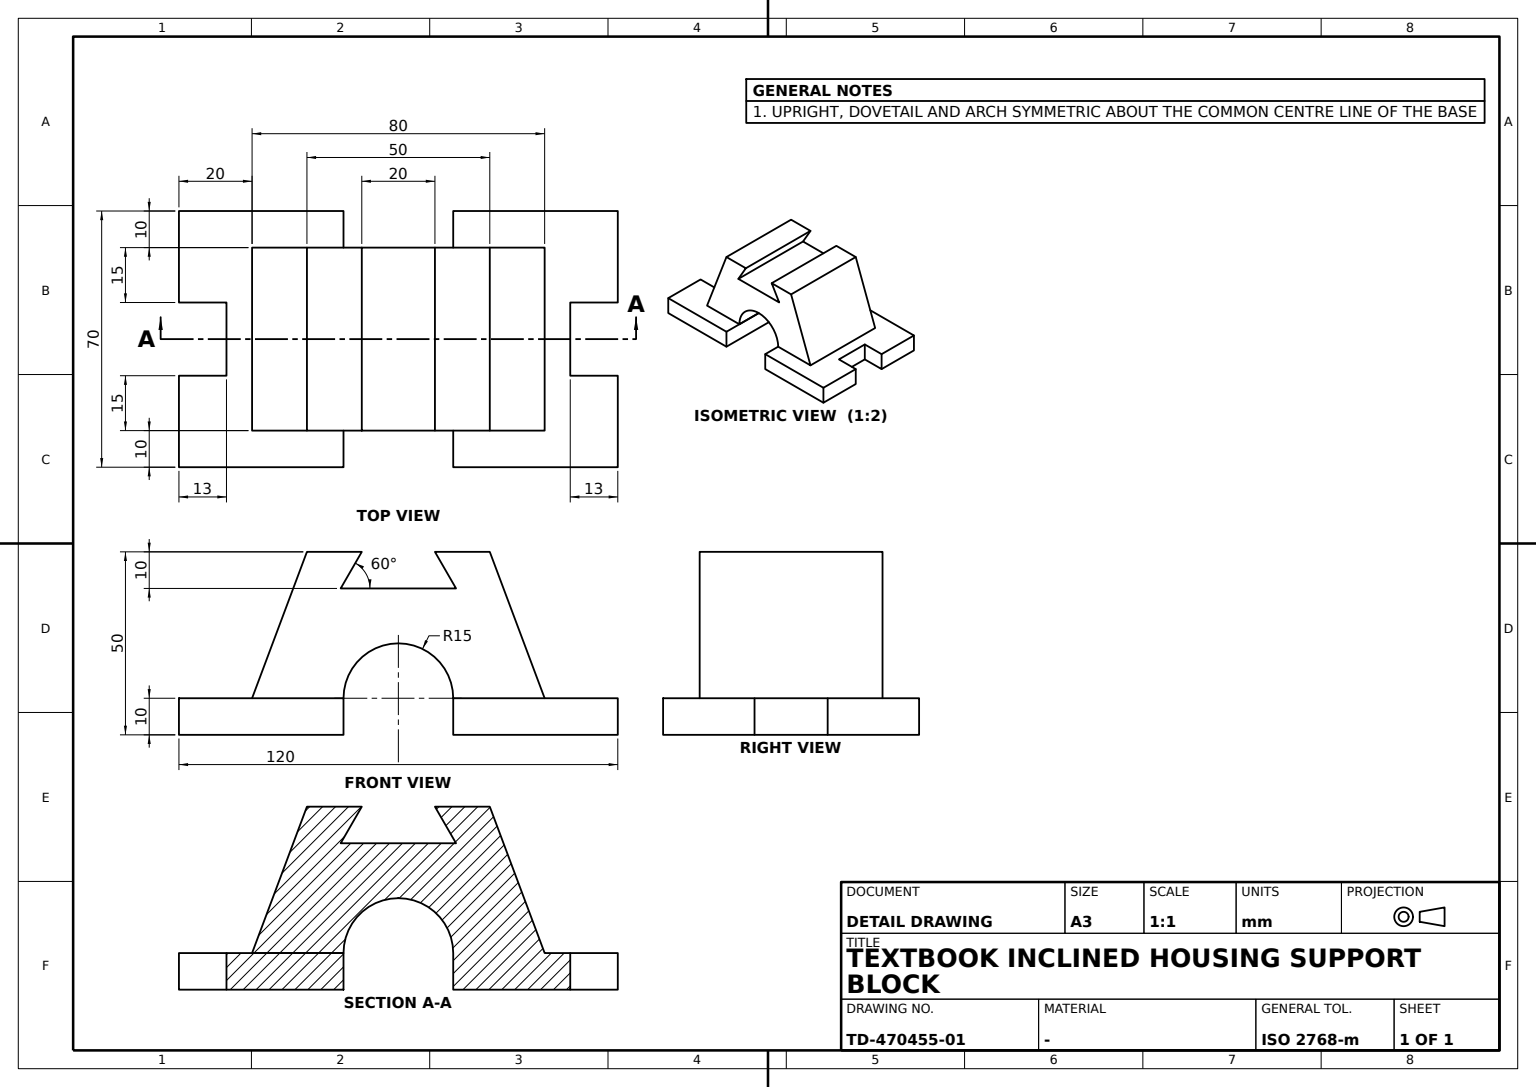
ISO-10303-21;
HEADER;
FILE_DESCRIPTION((''),'2;1');
FILE_NAME('','',(''),(''),'','','');
FILE_SCHEMA(('AUTOMOTIVE_DESIGN'));
ENDSEC;
DATA;
#1=APPLICATION_CONTEXT('');
#2=PRODUCT_CONTEXT('',#1,'mechanical');
#3=PRODUCT('','','',(#2));
#4=PRODUCT_DEFINITION_FORMATION('','',#3);
#5=PRODUCT_DEFINITION_CONTEXT('',#1,'design');
#6=PRODUCT_DEFINITION('','',#4,#5);
#7=PRODUCT_DEFINITION_SHAPE('','',#6);
#8=(LENGTH_UNIT()NAMED_UNIT(*)SI_UNIT(.MILLI.,.METRE.));
#9=(NAMED_UNIT(*)PLANE_ANGLE_UNIT()SI_UNIT($,.RADIAN.));
#10=(NAMED_UNIT(*)SI_UNIT($,.STERADIAN.)SOLID_ANGLE_UNIT());
#11=UNCERTAINTY_MEASURE_WITH_UNIT(LENGTH_MEASURE(0.005),#8,'distance_accuracy_value','');
#12=(GEOMETRIC_REPRESENTATION_CONTEXT(3)GLOBAL_UNCERTAINTY_ASSIGNED_CONTEXT((#11))GLOBAL_UNIT_ASSIGNED_CONTEXT((#8,#9,#10))REPRESENTATION_CONTEXT('',''));
#13=CARTESIAN_POINT('',(-15.773503,-25.,40.));
#14=VERTEX_POINT('',#13);
#15=CARTESIAN_POINT('',(15.773503,-25.,40.));
#16=VERTEX_POINT('',#15);
#17=DIRECTION('',(1.,0.,0.));
#18=VECTOR('',#17,1000.);
#19=LINE('',#13,#18);
#20=EDGE_CURVE('',#14,#16,#19,.T.);
#21=ORIENTED_EDGE('',*,*,#20,.T.);
#22=CARTESIAN_POINT('',(15.773503,25.,40.));
#23=VERTEX_POINT('',#22);
#24=DIRECTION('',(0.,1.,0.));
#25=VECTOR('',#24,1000.);
#26=LINE('',#22,#25);
#27=EDGE_CURVE('',#16,#23,#26,.T.);
#28=ORIENTED_EDGE('',*,*,#27,.T.);
#29=CARTESIAN_POINT('',(-15.773503,25.,40.));
#30=VERTEX_POINT('',#29);
#31=LINE('',#29,#18);
#32=EDGE_CURVE('',#30,#23,#31,.T.);
#33=ORIENTED_EDGE('',*,*,#32,.F.);
#34=LINE('',#29,#25);
#35=EDGE_CURVE('',#14,#30,#34,.T.);
#36=ORIENTED_EDGE('',*,*,#35,.F.);
#37=EDGE_LOOP('',(#21,#28,#33,#36));
#38=FACE_BOUND('',#37,.T.);
#39=DIRECTION('',(0.,0.,-1.));
#40=DIRECTION('',(-1.,0.,0.));
#41=AXIS2_PLACEMENT_3D('',#29,#39,#40);
#42=PLANE('',#41);
#43=ADVANCED_FACE('',(#38),#42,.F.);
#44=CARTESIAN_POINT('',(10.,25.,50.));
#45=VERTEX_POINT('',#44);
#46=CARTESIAN_POINT('',(10.,-25.,50.));
#47=VERTEX_POINT('',#46);
#48=DIRECTION('',(0.,-1.,0.));
#49=VECTOR('',#48,1000.);
#50=LINE('',#44,#49);
#51=EDGE_CURVE('',#45,#47,#50,.T.);
#52=ORIENTED_EDGE('',*,*,#51,.F.);
#53=DIRECTION('',(-0.5,0.,0.866025404));
#54=VECTOR('',#53,1000.);
#55=LINE('',#22,#54);
#56=EDGE_CURVE('',#23,#45,#55,.T.);
#57=ORIENTED_EDGE('',*,*,#56,.F.);
#58=ORIENTED_EDGE('',*,*,#27,.F.);
#59=LINE('',#15,#54);
#60=EDGE_CURVE('',#16,#47,#59,.T.);
#61=ORIENTED_EDGE('',*,*,#60,.T.);
#62=EDGE_LOOP('',(#52,#57,#58,#61));
#63=FACE_BOUND('',#62,.T.);
#64=DIRECTION('',(0.866025404,0.,0.5));
#65=DIRECTION('',(0.5,0.,-0.866025404));
#66=AXIS2_PLACEMENT_3D('',#22,#64,#65);
#67=PLANE('',#66);
#68=ADVANCED_FACE('',(#63),#67,.F.);
#69=CARTESIAN_POINT('',(40.,25.,10.));
#70=VERTEX_POINT('',#69);
#71=CARTESIAN_POINT('',(25.,25.,50.));
#72=VERTEX_POINT('',#71);
#73=DIRECTION('',(-0.351123442,0.,0.936329178));
#74=VECTOR('',#73,1000.);
#75=LINE('',#69,#74);
#76=EDGE_CURVE('',#70,#72,#75,.T.);
#77=ORIENTED_EDGE('',*,*,#76,.T.);
#78=CARTESIAN_POINT('',(25.,-25.,50.));
#79=VERTEX_POINT('',#78);
#80=LINE('',#78,#25);
#81=EDGE_CURVE('',#79,#72,#80,.T.);
#82=ORIENTED_EDGE('',*,*,#81,.F.);
#83=CARTESIAN_POINT('',(40.,-25.,10.));
#84=VERTEX_POINT('',#83);
#85=LINE('',#83,#74);
#86=EDGE_CURVE('',#84,#79,#85,.T.);
#87=ORIENTED_EDGE('',*,*,#86,.F.);
#88=LINE('',#83,#25);
#89=EDGE_CURVE('',#84,#70,#88,.T.);
#90=ORIENTED_EDGE('',*,*,#89,.T.);
#91=EDGE_LOOP('',(#77,#82,#87,#90));
#92=FACE_BOUND('',#91,.T.);
#93=DIRECTION('',(-0.936329178,0.,-0.351123442));
#94=AXIS2_PLACEMENT_3D('',#83,#93,#73);
#95=PLANE('',#94);
#96=ADVANCED_FACE('',(#92),#95,.F.);
#97=ORIENTED_EDGE('',*,*,#20,.F.);
#98=CARTESIAN_POINT('',(-10.,-25.,50.));
#99=VERTEX_POINT('',#98);
#100=DIRECTION('',(-0.5,0.,-0.866025404));
#101=VECTOR('',#100,1000.);
#102=LINE('',#98,#101);
#103=EDGE_CURVE('',#99,#14,#102,.T.);
#104=ORIENTED_EDGE('',*,*,#103,.F.);
#105=CARTESIAN_POINT('',(-25.,-25.,50.));
#106=VERTEX_POINT('',#105);
#107=VECTOR('',#40,1000.);
#108=LINE('',#78,#107);
#109=EDGE_CURVE('',#99,#106,#108,.T.);
#110=ORIENTED_EDGE('',*,*,#109,.T.);
#111=CARTESIAN_POINT('',(-40.,-25.,10.));
#112=VERTEX_POINT('',#111);
#113=DIRECTION('',(-0.351123442,0.,-0.936329178));
#114=VECTOR('',#113,1000.);
#115=LINE('',#105,#114);
#116=EDGE_CURVE('',#106,#112,#115,.T.);
#117=ORIENTED_EDGE('',*,*,#116,.T.);
#118=CARTESIAN_POINT('',(-15.,-25.,10.));
#119=VERTEX_POINT('',#118);
#120=LINE('',#111,#18);
#121=EDGE_CURVE('',#112,#119,#120,.T.);
#122=ORIENTED_EDGE('',*,*,#121,.T.);
#123=CARTESIAN_POINT('',(0.,-25.,25.));
#124=VERTEX_POINT('',#123);
#125=CARTESIAN_POINT('',(0.,-25.,10.));
#126=AXIS2_PLACEMENT_3D('',#125,#24,#17);
#127=CIRCLE('',#126,15.);
#128=EDGE_CURVE('',#119,#124,#127,.T.);
#129=ORIENTED_EDGE('',*,*,#128,.T.);
#130=CARTESIAN_POINT('',(15.,-25.,10.));
#131=VERTEX_POINT('',#130);
#132=EDGE_CURVE('',#124,#131,#127,.T.);
#133=ORIENTED_EDGE('',*,*,#132,.T.);
#134=LINE('',#130,#18);
#135=EDGE_CURVE('',#131,#84,#134,.T.);
#136=ORIENTED_EDGE('',*,*,#135,.T.);
#137=ORIENTED_EDGE('',*,*,#86,.T.);
#138=EDGE_CURVE('',#79,#47,#108,.T.);
#139=ORIENTED_EDGE('',*,*,#138,.T.);
#140=ORIENTED_EDGE('',*,*,#60,.F.);
#141=EDGE_LOOP('',(#97,#104,#110,#117,#122,#129,#133,#136,#137,#139,#140));
#142=FACE_BOUND('',#141,.T.);
#143=DIRECTION('',(0.,0.,1.));
#144=AXIS2_PLACEMENT_3D('',#125,#24,#143);
#145=PLANE('',#144);
#146=ADVANCED_FACE('',(#142),#145,.F.);
#147=CARTESIAN_POINT('',(-10.,25.,50.));
#148=VERTEX_POINT('',#147);
#149=LINE('',#147,#49);
#150=EDGE_CURVE('',#148,#99,#149,.T.);
#151=ORIENTED_EDGE('',*,*,#150,.T.);
#152=ORIENTED_EDGE('',*,*,#103,.T.);
#153=ORIENTED_EDGE('',*,*,#35,.T.);
#154=LINE('',#147,#101);
#155=EDGE_CURVE('',#148,#30,#154,.T.);
#156=ORIENTED_EDGE('',*,*,#155,.F.);
#157=EDGE_LOOP('',(#151,#152,#153,#156));
#158=FACE_BOUND('',#157,.T.);
#159=DIRECTION('',(-0.866025404,0.,0.5));
#160=DIRECTION('',(0.5,0.,0.866025404));
#161=AXIS2_PLACEMENT_3D('',#147,#159,#160);
#162=PLANE('',#161);
#163=ADVANCED_FACE('',(#158),#162,.F.);
#164=CARTESIAN_POINT('',(60.,10.,0.));
#165=VERTEX_POINT('',#164);
#166=CARTESIAN_POINT('',(60.,35.,0.));
#167=VERTEX_POINT('',#166);
#168=CARTESIAN_POINT('',(60.,-35.,0.));
#169=LINE('',#168,#25);
#170=EDGE_CURVE('',#165,#167,#169,.T.);
#171=ORIENTED_EDGE('',*,*,#170,.F.);
#172=CARTESIAN_POINT('',(47.,10.,0.));
#173=VERTEX_POINT('',#172);
#174=LINE('',#164,#107);
#175=EDGE_CURVE('',#165,#173,#174,.T.);
#176=ORIENTED_EDGE('',*,*,#175,.T.);
#177=CARTESIAN_POINT('',(47.,-10.,0.));
#178=VERTEX_POINT('',#177);
#179=LINE('',#172,#49);
#180=EDGE_CURVE('',#173,#178,#179,.T.);
#181=ORIENTED_EDGE('',*,*,#180,.T.);
#182=CARTESIAN_POINT('',(60.,-10.,0.));
#183=VERTEX_POINT('',#182);
#184=LINE('',#177,#18);
#185=EDGE_CURVE('',#178,#183,#184,.T.);
#186=ORIENTED_EDGE('',*,*,#185,.T.);
#187=VERTEX_POINT('',#168);
#188=EDGE_CURVE('',#187,#183,#169,.T.);
#189=ORIENTED_EDGE('',*,*,#188,.F.);
#190=CARTESIAN_POINT('',(15.,-35.,0.));
#191=VERTEX_POINT('',#190);
#192=CARTESIAN_POINT('',(-60.,-35.,0.));
#193=LINE('',#192,#18);
#194=EDGE_CURVE('',#191,#187,#193,.T.);
#195=ORIENTED_EDGE('',*,*,#194,.F.);
#196=CARTESIAN_POINT('',(15.,35.,0.));
#197=VERTEX_POINT('',#196);
#198=LINE('',#190,#25);
#199=EDGE_CURVE('',#191,#197,#198,.T.);
#200=ORIENTED_EDGE('',*,*,#199,.T.);
#201=LINE('',#166,#107);
#202=EDGE_CURVE('',#167,#197,#201,.T.);
#203=ORIENTED_EDGE('',*,*,#202,.F.);
#204=EDGE_LOOP('',(#171,#176,#181,#186,#189,#195,#200,#203));
#205=FACE_BOUND('',#204,.T.);
#206=CARTESIAN_POINT('',(0.,0.,0.));
#207=AXIS2_PLACEMENT_3D('',#206,#143,#17);
#208=PLANE('',#207);
#209=ADVANCED_FACE('',(#205),#208,.F.);
#210=CARTESIAN_POINT('',(-25.,25.,50.));
#211=VERTEX_POINT('',#210);
#212=CARTESIAN_POINT('',(-40.,25.,10.));
#213=VERTEX_POINT('',#212);
#214=LINE('',#210,#114);
#215=EDGE_CURVE('',#211,#213,#214,.T.);
#216=ORIENTED_EDGE('',*,*,#215,.F.);
#217=LINE('',#71,#107);
#218=EDGE_CURVE('',#148,#211,#217,.T.);
#219=ORIENTED_EDGE('',*,*,#218,.F.);
#220=ORIENTED_EDGE('',*,*,#155,.T.);
#221=ORIENTED_EDGE('',*,*,#32,.T.);
#222=ORIENTED_EDGE('',*,*,#56,.T.);
#223=EDGE_CURVE('',#72,#45,#217,.T.);
#224=ORIENTED_EDGE('',*,*,#223,.F.);
#225=ORIENTED_EDGE('',*,*,#76,.F.);
#226=CARTESIAN_POINT('',(15.,25.,10.));
#227=VERTEX_POINT('',#226);
#228=LINE('',#226,#18);
#229=EDGE_CURVE('',#227,#70,#228,.T.);
#230=ORIENTED_EDGE('',*,*,#229,.F.);
#231=CARTESIAN_POINT('',(0.,25.,25.));
#232=VERTEX_POINT('',#231);
#233=CARTESIAN_POINT('',(0.,25.,10.));
#234=AXIS2_PLACEMENT_3D('',#233,#24,#17);
#235=CIRCLE('',#234,15.);
#236=EDGE_CURVE('',#232,#227,#235,.T.);
#237=ORIENTED_EDGE('',*,*,#236,.F.);
#238=CARTESIAN_POINT('',(-15.,25.,10.));
#239=VERTEX_POINT('',#238);
#240=EDGE_CURVE('',#239,#232,#235,.T.);
#241=ORIENTED_EDGE('',*,*,#240,.F.);
#242=LINE('',#212,#18);
#243=EDGE_CURVE('',#213,#239,#242,.T.);
#244=ORIENTED_EDGE('',*,*,#243,.F.);
#245=EDGE_LOOP('',(#216,#219,#220,#221,#222,#224,#225,#230,#237,#241,#244));
#246=FACE_BOUND('',#245,.T.);
#247=AXIS2_PLACEMENT_3D('',#233,#24,#143);
#248=PLANE('',#247);
#249=ADVANCED_FACE('',(#246),#248,.T.);
#250=CARTESIAN_POINT('',(47.,-10.,10.));
#251=VERTEX_POINT('',#250);
#252=VECTOR('',#39,1000.);
#253=LINE('',#177,#252);
#254=EDGE_CURVE('',#251,#178,#253,.T.);
#255=ORIENTED_EDGE('',*,*,#254,.T.);
#256=ORIENTED_EDGE('',*,*,#180,.F.);
#257=CARTESIAN_POINT('',(47.,10.,10.));
#258=VERTEX_POINT('',#257);
#259=LINE('',#172,#252);
#260=EDGE_CURVE('',#258,#173,#259,.T.);
#261=ORIENTED_EDGE('',*,*,#260,.F.);
#262=LINE('',#257,#49);
#263=EDGE_CURVE('',#258,#251,#262,.T.);
#264=ORIENTED_EDGE('',*,*,#263,.T.);
#265=EDGE_LOOP('',(#255,#256,#261,#264));
#266=FACE_BOUND('',#265,.T.);
#267=AXIS2_PLACEMENT_3D('',#172,#40,#143);
#268=PLANE('',#267);
#269=ADVANCED_FACE('',(#266),#268,.F.);
#270=CARTESIAN_POINT('',(60.,35.,10.));
#271=VERTEX_POINT('',#270);
#272=LINE('',#270,#252);
#273=EDGE_CURVE('',#271,#167,#272,.T.);
#274=ORIENTED_EDGE('',*,*,#273,.T.);
#275=ORIENTED_EDGE('',*,*,#202,.T.);
#276=CARTESIAN_POINT('',(15.,35.,10.));
#277=VERTEX_POINT('',#276);
#278=VECTOR('',#143,1000.);
#279=LINE('',#196,#278);
#280=EDGE_CURVE('',#197,#277,#279,.T.);
#281=ORIENTED_EDGE('',*,*,#280,.T.);
#282=LINE('',#270,#107);
#283=EDGE_CURVE('',#271,#277,#282,.T.);
#284=ORIENTED_EDGE('',*,*,#283,.F.);
#285=EDGE_LOOP('',(#274,#275,#281,#284));
#286=FACE_BOUND('',#285,.T.);
#287=AXIS2_PLACEMENT_3D('',#270,#48,#39);
#288=PLANE('',#287);
#289=ADVANCED_FACE('',(#286),#288,.F.);
#290=CARTESIAN_POINT('',(15.,-35.,10.));
#291=VERTEX_POINT('',#290);
#292=CARTESIAN_POINT('',(60.,-35.,10.));
#293=VERTEX_POINT('',#292);
#294=CARTESIAN_POINT('',(-60.,-35.,10.));
#295=LINE('',#294,#18);
#296=EDGE_CURVE('',#291,#293,#295,.T.);
#297=ORIENTED_EDGE('',*,*,#296,.T.);
#298=CARTESIAN_POINT('',(60.,-10.,10.));
#299=VERTEX_POINT('',#298);
#300=LINE('',#292,#25);
#301=EDGE_CURVE('',#293,#299,#300,.T.);
#302=ORIENTED_EDGE('',*,*,#301,.T.);
#303=LINE('',#250,#18);
#304=EDGE_CURVE('',#251,#299,#303,.T.);
#305=ORIENTED_EDGE('',*,*,#304,.F.);
#306=ORIENTED_EDGE('',*,*,#263,.F.);
#307=CARTESIAN_POINT('',(60.,10.,10.));
#308=VERTEX_POINT('',#307);
#309=LINE('',#307,#107);
#310=EDGE_CURVE('',#308,#258,#309,.T.);
#311=ORIENTED_EDGE('',*,*,#310,.F.);
#312=EDGE_CURVE('',#308,#271,#300,.T.);
#313=ORIENTED_EDGE('',*,*,#312,.T.);
#314=ORIENTED_EDGE('',*,*,#283,.T.);
#315=LINE('',#290,#25);
#316=EDGE_CURVE('',#227,#277,#315,.T.);
#317=ORIENTED_EDGE('',*,*,#316,.F.);
#318=ORIENTED_EDGE('',*,*,#229,.T.);
#319=ORIENTED_EDGE('',*,*,#89,.F.);
#320=ORIENTED_EDGE('',*,*,#135,.F.);
#321=EDGE_CURVE('',#291,#131,#315,.T.);
#322=ORIENTED_EDGE('',*,*,#321,.F.);
#323=EDGE_LOOP('',(#297,#302,#305,#306,#311,#313,#314,#317,#318,#319,#320,#322));
#324=FACE_BOUND('',#323,.T.);
#325=CARTESIAN_POINT('',(0.,0.,10.));
#326=AXIS2_PLACEMENT_3D('',#325,#143,#17);
#327=PLANE('',#326);
#328=ADVANCED_FACE('',(#324),#327,.T.);
#329=ORIENTED_EDGE('',*,*,#81,.T.);
#330=ORIENTED_EDGE('',*,*,#223,.T.);
#331=ORIENTED_EDGE('',*,*,#51,.T.);
#332=ORIENTED_EDGE('',*,*,#138,.F.);
#333=EDGE_LOOP('',(#329,#330,#331,#332));
#334=FACE_BOUND('',#333,.T.);
#335=AXIS2_PLACEMENT_3D('',#78,#39,#40);
#336=PLANE('',#335);
#337=ADVANCED_FACE('',(#334),#336,.F.);
#338=ORIENTED_EDGE('',*,*,#199,.F.);
#339=LINE('',#190,#278);
#340=EDGE_CURVE('',#191,#291,#339,.T.);
#341=ORIENTED_EDGE('',*,*,#340,.T.);
#342=ORIENTED_EDGE('',*,*,#321,.T.);
#343=LINE('',#130,#25);
#344=EDGE_CURVE('',#131,#227,#343,.T.);
#345=ORIENTED_EDGE('',*,*,#344,.T.);
#346=ORIENTED_EDGE('',*,*,#316,.T.);
#347=ORIENTED_EDGE('',*,*,#280,.F.);
#348=EDGE_LOOP('',(#338,#341,#342,#345,#346,#347));
#349=FACE_BOUND('',#348,.T.);
#350=AXIS2_PLACEMENT_3D('',#190,#17,#24);
#351=PLANE('',#350);
#352=ADVANCED_FACE('',(#349),#351,.F.);
#353=LINE('',#118,#25);
#354=EDGE_CURVE('',#119,#239,#353,.T.);
#355=ORIENTED_EDGE('',*,*,#354,.T.);
#356=ORIENTED_EDGE('',*,*,#240,.T.);
#357=LINE('',#123,#25);
#358=EDGE_CURVE('',#124,#232,#357,.T.);
#359=ORIENTED_EDGE('',*,*,#358,.F.);
#360=ORIENTED_EDGE('',*,*,#128,.F.);
#361=EDGE_LOOP('',(#355,#356,#359,#360));
#362=FACE_BOUND('',#361,.T.);
#363=CYLINDRICAL_SURFACE('',#144,15.);
#364=ADVANCED_FACE('',(#362),#363,.F.);
#365=ORIENTED_EDGE('',*,*,#273,.F.);
#366=ORIENTED_EDGE('',*,*,#312,.F.);
#367=LINE('',#164,#278);
#368=EDGE_CURVE('',#165,#308,#367,.T.);
#369=ORIENTED_EDGE('',*,*,#368,.F.);
#370=ORIENTED_EDGE('',*,*,#170,.T.);
#371=EDGE_LOOP('',(#365,#366,#369,#370));
#372=FACE_BOUND('',#371,.T.);
#373=AXIS2_PLACEMENT_3D('',#292,#40,#48);
#374=PLANE('',#373);
#375=ADVANCED_FACE('',(#372),#374,.F.);
#376=ORIENTED_EDGE('',*,*,#121,.F.);
#377=LINE('',#111,#25);
#378=EDGE_CURVE('',#112,#213,#377,.T.);
#379=ORIENTED_EDGE('',*,*,#378,.T.);
#380=ORIENTED_EDGE('',*,*,#243,.T.);
#381=ORIENTED_EDGE('',*,*,#354,.F.);
#382=EDGE_LOOP('',(#376,#379,#380,#381));
#383=FACE_BOUND('',#382,.T.);
#384=AXIS2_PLACEMENT_3D('',#111,#143,#17);
#385=PLANE('',#384);
#386=ADVANCED_FACE('',(#383),#385,.F.);
#387=ORIENTED_EDGE('',*,*,#344,.F.);
#388=ORIENTED_EDGE('',*,*,#132,.F.);
#389=ORIENTED_EDGE('',*,*,#358,.T.);
#390=ORIENTED_EDGE('',*,*,#236,.T.);
#391=EDGE_LOOP('',(#387,#388,#389,#390));
#392=FACE_BOUND('',#391,.T.);
#393=ADVANCED_FACE('',(#392),#363,.F.);
#394=ORIENTED_EDGE('',*,*,#175,.F.);
#395=ORIENTED_EDGE('',*,*,#368,.T.);
#396=ORIENTED_EDGE('',*,*,#310,.T.);
#397=ORIENTED_EDGE('',*,*,#260,.T.);
#398=EDGE_LOOP('',(#394,#395,#396,#397));
#399=FACE_BOUND('',#398,.T.);
#400=AXIS2_PLACEMENT_3D('',#164,#24,#40);
#401=PLANE('',#400);
#402=ADVANCED_FACE('',(#399),#401,.F.);
#403=LINE('',#182,#278);
#404=EDGE_CURVE('',#183,#299,#403,.T.);
#405=ORIENTED_EDGE('',*,*,#404,.T.);
#406=ORIENTED_EDGE('',*,*,#301,.F.);
#407=LINE('',#292,#252);
#408=EDGE_CURVE('',#293,#187,#407,.T.);
#409=ORIENTED_EDGE('',*,*,#408,.T.);
#410=ORIENTED_EDGE('',*,*,#188,.T.);
#411=EDGE_LOOP('',(#405,#406,#409,#410));
#412=FACE_BOUND('',#411,.T.);
#413=ADVANCED_FACE('',(#412),#374,.F.);
#414=ORIENTED_EDGE('',*,*,#340,.F.);
#415=ORIENTED_EDGE('',*,*,#194,.T.);
#416=ORIENTED_EDGE('',*,*,#408,.F.);
#417=ORIENTED_EDGE('',*,*,#296,.F.);
#418=EDGE_LOOP('',(#414,#415,#416,#417));
#419=FACE_BOUND('',#418,.T.);
#420=AXIS2_PLACEMENT_3D('',#294,#24,#143);
#421=PLANE('',#420);
#422=ADVANCED_FACE('',(#419),#421,.F.);
#423=ORIENTED_EDGE('',*,*,#304,.T.);
#424=ORIENTED_EDGE('',*,*,#404,.F.);
#425=ORIENTED_EDGE('',*,*,#185,.F.);
#426=ORIENTED_EDGE('',*,*,#254,.F.);
#427=EDGE_LOOP('',(#423,#424,#425,#426));
#428=FACE_BOUND('',#427,.T.);
#429=AXIS2_PLACEMENT_3D('',#177,#48,#17);
#430=PLANE('',#429);
#431=ADVANCED_FACE('',(#428),#430,.F.);
#432=ORIENTED_EDGE('',*,*,#116,.F.);
#433=LINE('',#105,#25);
#434=EDGE_CURVE('',#106,#211,#433,.T.);
#435=ORIENTED_EDGE('',*,*,#434,.T.);
#436=ORIENTED_EDGE('',*,*,#215,.T.);
#437=ORIENTED_EDGE('',*,*,#378,.F.);
#438=EDGE_LOOP('',(#432,#435,#436,#437));
#439=FACE_BOUND('',#438,.T.);
#440=DIRECTION('',(0.936329178,0.,-0.351123442));
#441=AXIS2_PLACEMENT_3D('',#105,#440,#113);
#442=PLANE('',#441);
#443=ADVANCED_FACE('',(#439),#442,.F.);
#444=ORIENTED_EDGE('',*,*,#109,.F.);
#445=ORIENTED_EDGE('',*,*,#150,.F.);
#446=ORIENTED_EDGE('',*,*,#218,.T.);
#447=ORIENTED_EDGE('',*,*,#434,.F.);
#448=EDGE_LOOP('',(#444,#445,#446,#447));
#449=FACE_BOUND('',#448,.T.);
#450=ADVANCED_FACE('',(#449),#336,.F.);
#451=CLOSED_SHELL('',(#43,#68,#96,#146,#163,#209,#249,#269,#289,#328,#337,#352,#364,#375,#386,#393,#402,#413,#422,#431,#443,#450));
#452=MANIFOLD_SOLID_BREP('',#451);
#453=VERTEX_POINT('',#294);
#454=CARTESIAN_POINT('',(-15.,-35.,10.));
#455=VERTEX_POINT('',#454);
#456=EDGE_CURVE('',#453,#455,#295,.T.);
#457=ORIENTED_EDGE('',*,*,#456,.F.);
#458=VERTEX_POINT('',#192);
#459=LINE('',#294,#252);
#460=EDGE_CURVE('',#453,#458,#459,.T.);
#461=ORIENTED_EDGE('',*,*,#460,.T.);
#462=CARTESIAN_POINT('',(-15.,-35.,0.));
#463=VERTEX_POINT('',#462);
#464=EDGE_CURVE('',#458,#463,#193,.T.);
#465=ORIENTED_EDGE('',*,*,#464,.T.);
#466=LINE('',#462,#278);
#467=EDGE_CURVE('',#463,#455,#466,.T.);
#468=ORIENTED_EDGE('',*,*,#467,.T.);
#469=EDGE_LOOP('',(#457,#461,#465,#468));
#470=FACE_BOUND('',#469,.T.);
#471=ADVANCED_FACE('',(#470),#421,.F.);
#472=ORIENTED_EDGE('',*,*,#460,.F.);
#473=CARTESIAN_POINT('',(-60.,-10.,10.));
#474=VERTEX_POINT('',#473);
#475=CARTESIAN_POINT('',(-60.,35.,10.));
#476=LINE('',#475,#49);
#477=EDGE_CURVE('',#474,#453,#476,.T.);
#478=ORIENTED_EDGE('',*,*,#477,.F.);
#479=CARTESIAN_POINT('',(-60.,-10.,0.));
#480=VERTEX_POINT('',#479);
#481=LINE('',#479,#278);
#482=EDGE_CURVE('',#480,#474,#481,.T.);
#483=ORIENTED_EDGE('',*,*,#482,.F.);
#484=CARTESIAN_POINT('',(-60.,35.,0.));
#485=LINE('',#484,#49);
#486=EDGE_CURVE('',#480,#458,#485,.T.);
#487=ORIENTED_EDGE('',*,*,#486,.T.);
#488=EDGE_LOOP('',(#472,#478,#483,#487));
#489=FACE_BOUND('',#488,.T.);
#490=AXIS2_PLACEMENT_3D('',#475,#17,#24);
#491=PLANE('',#490);
#492=ADVANCED_FACE('',(#489),#491,.F.);
#493=CARTESIAN_POINT('',(-47.,10.,10.));
#494=VERTEX_POINT('',#493);
#495=CARTESIAN_POINT('',(-60.,10.,10.));
#496=VERTEX_POINT('',#495);
#497=LINE('',#493,#107);
#498=EDGE_CURVE('',#494,#496,#497,.T.);
#499=ORIENTED_EDGE('',*,*,#498,.F.);
#500=CARTESIAN_POINT('',(-47.,-10.,10.));
#501=VERTEX_POINT('',#500);
#502=LINE('',#500,#25);
#503=EDGE_CURVE('',#501,#494,#502,.T.);
#504=ORIENTED_EDGE('',*,*,#503,.F.);
#505=LINE('',#473,#18);
#506=EDGE_CURVE('',#474,#501,#505,.T.);
#507=ORIENTED_EDGE('',*,*,#506,.F.);
#508=ORIENTED_EDGE('',*,*,#477,.T.);
#509=ORIENTED_EDGE('',*,*,#456,.T.);
#510=CARTESIAN_POINT('',(-15.,35.,10.));
#511=VERTEX_POINT('',#510);
#512=LINE('',#510,#49);
#513=EDGE_CURVE('',#511,#455,#512,.T.);
#514=ORIENTED_EDGE('',*,*,#513,.F.);
#515=VERTEX_POINT('',#475);
#516=EDGE_CURVE('',#511,#515,#282,.T.);
#517=ORIENTED_EDGE('',*,*,#516,.T.);
#518=EDGE_CURVE('',#515,#496,#476,.T.);
#519=ORIENTED_EDGE('',*,*,#518,.T.);
#520=EDGE_LOOP('',(#499,#504,#507,#508,#509,#514,#517,#519));
#521=FACE_BOUND('',#520,.T.);
#522=ADVANCED_FACE('',(#521),#327,.T.);
#523=ORIENTED_EDGE('',*,*,#513,.T.);
#524=ORIENTED_EDGE('',*,*,#467,.F.);
#525=CARTESIAN_POINT('',(-15.,35.,0.));
#526=VERTEX_POINT('',#525);
#527=LINE('',#525,#49);
#528=EDGE_CURVE('',#526,#463,#527,.T.);
#529=ORIENTED_EDGE('',*,*,#528,.F.);
#530=LINE('',#525,#278);
#531=EDGE_CURVE('',#526,#511,#530,.T.);
#532=ORIENTED_EDGE('',*,*,#531,.T.);
#533=EDGE_LOOP('',(#523,#524,#529,#532));
#534=FACE_BOUND('',#533,.T.);
#535=AXIS2_PLACEMENT_3D('',#525,#40,#48);
#536=PLANE('',#535);
#537=ADVANCED_FACE('',(#534),#536,.F.);
#538=CARTESIAN_POINT('',(-47.,10.,0.));
#539=VERTEX_POINT('',#538);
#540=LINE('',#538,#252);
#541=EDGE_CURVE('',#494,#539,#540,.T.);
#542=ORIENTED_EDGE('',*,*,#541,.T.);
#543=CARTESIAN_POINT('',(-47.,-10.,0.));
#544=VERTEX_POINT('',#543);
#545=LINE('',#543,#25);
#546=EDGE_CURVE('',#544,#539,#545,.T.);
#547=ORIENTED_EDGE('',*,*,#546,.F.);
#548=LINE('',#543,#252);
#549=EDGE_CURVE('',#501,#544,#548,.T.);
#550=ORIENTED_EDGE('',*,*,#549,.F.);
#551=ORIENTED_EDGE('',*,*,#503,.T.);
#552=EDGE_LOOP('',(#542,#547,#550,#551));
#553=FACE_BOUND('',#552,.T.);
#554=AXIS2_PLACEMENT_3D('',#543,#17,#39);
#555=PLANE('',#554);
#556=ADVANCED_FACE('',(#553),#555,.F.);
#557=CARTESIAN_POINT('',(-60.,10.,0.));
#558=VERTEX_POINT('',#557);
#559=LINE('',#557,#278);
#560=EDGE_CURVE('',#558,#496,#559,.T.);
#561=ORIENTED_EDGE('',*,*,#560,.T.);
#562=ORIENTED_EDGE('',*,*,#518,.F.);
#563=VERTEX_POINT('',#484);
#564=LINE('',#475,#252);
#565=EDGE_CURVE('',#515,#563,#564,.T.);
#566=ORIENTED_EDGE('',*,*,#565,.T.);
#567=EDGE_CURVE('',#563,#558,#485,.T.);
#568=ORIENTED_EDGE('',*,*,#567,.T.);
#569=EDGE_LOOP('',(#561,#562,#566,#568));
#570=FACE_BOUND('',#569,.T.);
#571=ADVANCED_FACE('',(#570),#491,.F.);
#572=ORIENTED_EDGE('',*,*,#506,.T.);
#573=ORIENTED_EDGE('',*,*,#549,.T.);
#574=LINE('',#479,#18);
#575=EDGE_CURVE('',#480,#544,#574,.T.);
#576=ORIENTED_EDGE('',*,*,#575,.F.);
#577=ORIENTED_EDGE('',*,*,#482,.T.);
#578=EDGE_LOOP('',(#572,#573,#576,#577));
#579=FACE_BOUND('',#578,.T.);
#580=AXIS2_PLACEMENT_3D('',#479,#48,#17);
#581=PLANE('',#580);
#582=ADVANCED_FACE('',(#579),#581,.F.);
#583=ORIENTED_EDGE('',*,*,#486,.F.);
#584=ORIENTED_EDGE('',*,*,#575,.T.);
#585=ORIENTED_EDGE('',*,*,#546,.T.);
#586=LINE('',#538,#107);
#587=EDGE_CURVE('',#539,#558,#586,.T.);
#588=ORIENTED_EDGE('',*,*,#587,.T.);
#589=ORIENTED_EDGE('',*,*,#567,.F.);
#590=EDGE_CURVE('',#526,#563,#201,.T.);
#591=ORIENTED_EDGE('',*,*,#590,.F.);
#592=ORIENTED_EDGE('',*,*,#528,.T.);
#593=ORIENTED_EDGE('',*,*,#464,.F.);
#594=EDGE_LOOP('',(#583,#584,#585,#588,#589,#591,#592,#593));
#595=FACE_BOUND('',#594,.T.);
#596=ADVANCED_FACE('',(#595),#208,.F.);
#597=ORIENTED_EDGE('',*,*,#516,.F.);
#598=ORIENTED_EDGE('',*,*,#531,.F.);
#599=ORIENTED_EDGE('',*,*,#590,.T.);
#600=ORIENTED_EDGE('',*,*,#565,.F.);
#601=EDGE_LOOP('',(#597,#598,#599,#600));
#602=FACE_BOUND('',#601,.T.);
#603=ADVANCED_FACE('',(#602),#288,.F.);
#604=ORIENTED_EDGE('',*,*,#541,.F.);
#605=ORIENTED_EDGE('',*,*,#498,.T.);
#606=ORIENTED_EDGE('',*,*,#560,.F.);
#607=ORIENTED_EDGE('',*,*,#587,.F.);
#608=EDGE_LOOP('',(#604,#605,#606,#607));
#609=FACE_BOUND('',#608,.T.);
#610=AXIS2_PLACEMENT_3D('',#538,#24,#40);
#611=PLANE('',#610);
#612=ADVANCED_FACE('',(#609),#611,.F.);
#613=CLOSED_SHELL('',(#471,#492,#522,#537,#556,#571,#582,#596,#603,#612));
#614=MANIFOLD_SOLID_BREP('',#613);
#615=ADVANCED_BREP_SHAPE_REPRESENTATION('',(#452,#614),#12);
#616=SHAPE_DEFINITION_REPRESENTATION(#7,#615);
ENDSEC;
END-ISO-10303-21;
